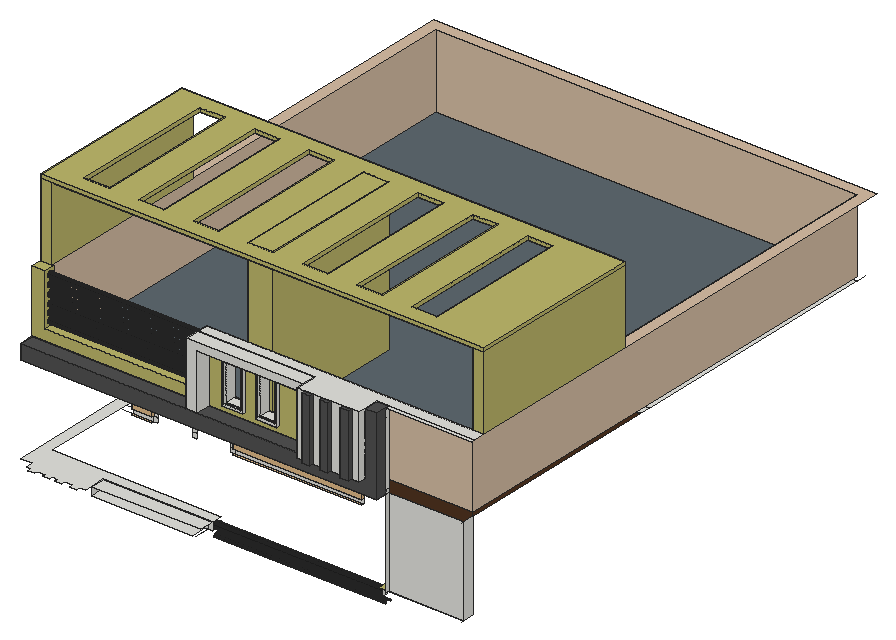
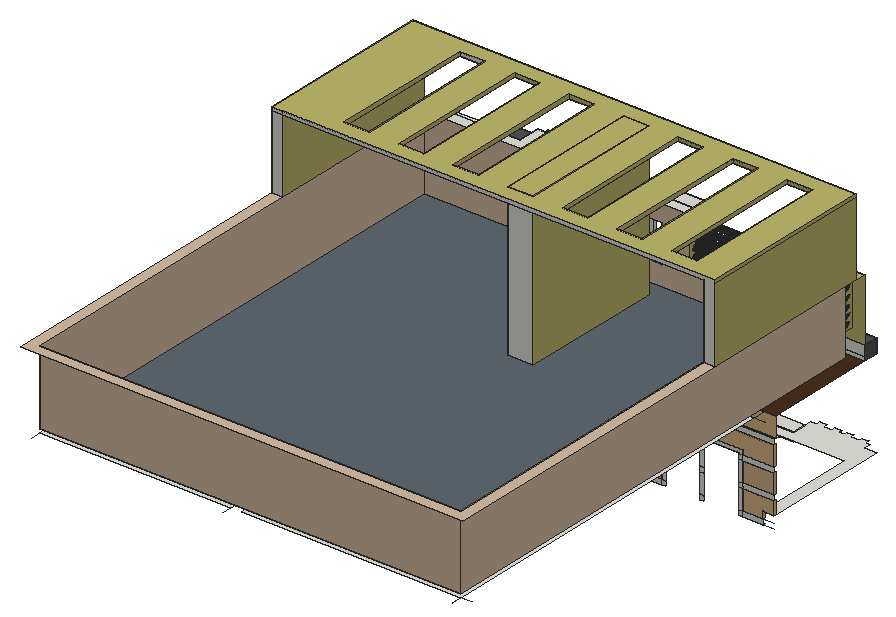
# SketchUp Ruby script. Lengths in inches.
U = 1.inch
M = Sketchup.active_model
def pt(a) = Geom::Point3d.new(a.map { |v| v * U })
def face(e, loops, mat)
  f = e.add_face(loops[0].map { |a| pt(a) })
  loops[1..].each { |l| e.add_face(l.map { |a| pt(a) }).erase! }
  f.material = f.back_material = mat if mat
  f
end
# faces: each face lists its corners as indices into pts; further lists are holes
def faces(e, pts, list, mat = nil) = list.each { |f| face(e, (f[0].is_a?(Array) ? f : [f]).map { |l| l.map { |i| pts[i] } }, mat) }
# xy, xz, yz: faces in a plane at the given z, y or x. An outline is a flat list of corners, or four numbers for a rectangle; further outlines are holes
def ring(l) = l.size == 4 ? [[l[0], l[1]], [l[2], l[1]], [l[2], l[3]], [l[0], l[3]]] : l.each_slice(2).to_a
def flat(e, list, mat, &to3) = list.each { |f| face(e, (f[0].is_a?(Array) ? f : [f]).map { |l| ring(l).map { |u, v| to3.(u, v) } }, mat) }
def xy(e, z, list, mat = nil) = flat(e, list, mat) { |x, y| [x, y, z] }
def xz(e, y, list, mat = nil) = flat(e, list, mat) { |x, z| [x, y, z] }
def yz(e, x, list, mat = nil) = flat(e, list, mat) { |y, z| [x, y, z] }
def lines(e, pts, list) = list.each { |a, b| e.add_line(pt(pts[a]), pt(pts[b])) }
# prism: a flat outline (further loops are holes) pulled along v
def prism(e, loops, v, mat = nil)
  f = face(e, loops, mat); d = Geom::Vector3d.new(v.map { |x| x * U })
  f.pushpull(f.normal.samedirection?(d) ? d.length : -d.length)
end
def box(e, o, s, mat = nil) = prism(e, [[o, [o[0] + s[0], o[1], o[2]], [o[0] + s[0], o[1] + s[1], o[2]], [o[0], o[1] + s[1], o[2]]]], [0, 0, s[2]], mat)
def at(x, y, z, deg = 0) = Geom::Transformation.translation(pt([x, y, z])) * Geom::Transformation.rotation(ORIGIN, Z_AXIS, deg.degrees)
def axes(o, x, y, z) = Geom::Transformation.new([*x, 0, *y, 0, *z, 0, *pt(o).to_a, 1])
def part(name) = M.definitions.add(name)
# library, detail: a bought-in or finely detailed component or shape, given as its bounding box
def library(name, o, s) = part(name).tap { |d| box(d.entities, o, s) }
def detail(e, o, s) = box(e.add_group.entities, o, s)
def put(e, d, t, mat = nil) = e.add_instance(d, t).tap { |i| i.material = mat if mat }
def group(e, t, mat = nil) = e.add_group.tap { |g| g.transformation = t; g.material = mat if mat }.entities
root = M.entities
M.materials.add("[0035_Tan]").color = [210, 180, 140]
M.materials.add("[0036_BurlyWood]").color = [222, 184, 135]
M.materials.add("[0043_SaddleBrown]2").color = [76, 37, 10]
M.materials.add("[0057_DarkKhaki]").color = [189, 183, 107]
M.materials.add("[0135_DarkGray]").color = [81, 81, 81]
M.materials.add("[Beadboard]").color = [71, 46, 29]
M.materials.add("[Blacktop New]").color = [30, 30, 30]
M.materials.add("[Formica Laminate Light]").color = [213, 189, 164]
M.materials.add("[Formica Speckled Grey]").color = [94, 105, 111]
M.materials.add("[Wood Veneer 01]").color = [120, 70, 37]
xy(root,281.25,[[9,110.875,25.44,112.875],[91.44,110.875,195.9375,112.875]],"[0036_BurlyWood]")
xy(root,282.05,[[70.9375,18,88.25,21],[104.5625,18,121.875,21]])
xy(root,284.36,[[57.8125,9,140.4375,21]])
xy(root,285.34,[[9,110.875,25.44,112.875],[91.44,110.875,195.9375,112.875]],"[0036_BurlyWood]")
xy(root,291,[[13.18,0,18.97,0,18.97,3,25.43,3,25.43,0,31.22,0,31.22,3,35.56,3,35.56,0,41.34,0,41.34,3,47.49,3,47.49,0,53.28,0,53.28,3,57.8125,3,57.8125,21,146.625,21,146.625,30,9,30,9,110.875,0,110.875,0,9,9.76,9,9.76,3,13.18,3],[57.8125,9,146.625,21]])
xy(root,291,[[0,110.875,9,112.875]],"[0036_BurlyWood]")
xy(root,291,[[282.375,21,351,30]],"[0057_DarkKhaki]")
xy(root,301.6875,[[0,110.875,9,112.875],[9,110.875,25.44,112.875],[91.44,110.875,195.9375,112.875]],"[0036_BurlyWood]")
xy(root,305.78,[[0,110.875,25.44,112.875]],"[0035_Tan]")
xy(root,305.78,[[91.44,110.875,195.9375,112.875]],"[0036_BurlyWood]")
xy(root,322.125,[[0,110.875,9,112.875],[9,110.875,25.44,112.875]],"[0035_Tan]")
xy(root,322.125,[[91.44,110.875,195.9375,112.875]],"[0036_BurlyWood]")
xy(root,326.22,[[0,110.875,25.44,112.875],[91.44,110.875,195.9375,112.875]],"[0036_BurlyWood]")
xy(root,327,[[28.44,109.875,57.44,112.875],[60.44,109.875,88.44,112.875],[230.67,198,254.61,201],[257.61,198,278.67,201]],"[0043_SaddleBrown]2")
xy(root,330,[[25.44,110.875,91.44,112.875]],"[0036_BurlyWood]")
xy(root,330,[[25.44,109.875,91.44,110.875]],"[0043_SaddleBrown]2")
xy(root,333,[[224.97,200,228.8125,201],[232.16,200,236,201],[239.34,200,243.1875,201],[246.53,200,250.375,201],[253.72,200,257.5625,201],
  [260.91,200,264.75,201],[268.09,200,271.9375,201],[275.28,200,279.125,201],[282.47,200,284.67,201]])
xy(root,333,[[224.67,198,284.67,198,284.67,200,282.47,200,282.47,201,279.125,201,279.125,200,275.28,200,275.28,201,271.9375,201,271.9375,200,268.09,200,268.09,201,264.75,201,264.75,200,260.91,200,260.91,201,257.5625,201,257.5625,200,253.72,200,253.72,201,250.375,201,250.375,200,246.53,200,246.53,201,243.1875,201,243.1875,200,239.34,200,239.34,201,236,201,236,200,232.16,200,232.16,201,228.8125,201,228.8125,200,224.97,200,224.97,201,224.67,201]],"[0043_SaddleBrown]2")
xy(root,342.5625,[[0,110.875,9,112.875],[9,110.875,195.9375,112.875]],"[0036_BurlyWood]")
xy(root,346.66,[[0,110.875,195.9375,112.875]],"[0036_BurlyWood]")
xy(root,363,[[9,121.875,186.9375,420],[196.22,200,200.0625,201],[203.41,200,207.25,201],[210.59,200,214.4375,201],[217.78,200,221.625,201],
  [224.97,200,228.8125,201],[232.16,200,236,201],[239.34,200,243.1875,201],[246.53,200,250.375,201],[253.72,200,257.5625,201],
  [260.91,200,264.75,201],[268.09,200,271.9375,201],[275.28,200,279.125,201],[282.47,200,286.3125,201],[289.66,200,293.5,201],
  [296.84,200,300.6875,201],[304.03,200,307.875,201],[311.22,200,315.0625,201],[318.41,200,322.25,201],[325.59,200,329.4375,201],
  [332.78,200,336.625,201],[339.97,200,343.8125,201],[347.16,200,351,201],[195.9375,201,351,210],[195.9375,210,351,420]])
xy(root,363,[[0,9,290.11,21]],"[0135_DarkGray]")
xy(root,363,[[0,21,0,110.875,195.9375,110.875,195.9375,201,196.22,201,196.22,200,200.0625,200,200.0625,201,203.41,201,203.41,200,207.25,200,207.25,201,210.59,201,210.59,200,214.4375,200,214.4375,201,217.78,201,217.78,200,221.625,200,221.625,201,224.97,201,224.97,200,228.8125,200,228.8125,201,232.16,201,232.16,200,236,200,236,201,239.34,201,239.34,200,243.1875,200,243.1875,201,246.53,201,246.53,200,250.375,200,250.375,201,253.72,201,253.72,200,257.5625,200,257.5625,201,260.91,201,260.91,200,264.75,200,264.75,201,268.09,201,268.09,200,271.9375,200,271.9375,201,275.28,201,275.28,200,279.125,200,279.125,201,282.47,201,282.47,200,286.3125,200,286.3125,201,289.66,201,289.66,200,293.5,200,293.5,201,296.84,201,296.84,200,300.6875,200,300.6875,201,304.03,201,304.03,200,307.875,200,307.875,201,311.22,201,311.22,200,315.0625,200,315.0625,201,318.41,201,318.41,200,322.25,200,322.25,201,325.59,201,325.59,200,329.4375,200,329.4375,201,332.78,201,332.78,200,336.625,200,336.625,201,339.97,201,339.97,200,343.8125,200,343.8125,201,347.16,201,347.16,200,351,200,351,21]],"[Beadboard]")
xy(root,366,[[[9,30,351,420],[157.91,43.02,178.34,160.52]]],"[Formica Speckled Grey]")
xy(root,374.8125,[[229.86,3,280.28,9],[229.86,9,280.28,21]])
xy(root,374.8125,[[235.76,0,242.96,3],[250.32,0,257.52,3],[266.89,0,274.09,3],[0,9,229.86,9,229.86,21,143.76,21,143.76,9.1875,134.73,9.1875,134.73,21,0,21]],"[0135_DarkGray]")
xy(root,379.88,[[155.82,19,173.26,21],[183.51,19,200.94,21]])
xy(root,381.88,[[157.82,19,171.26,21],[185.51,19,198.94,21],[157.82,21,171.26,30],[185.51,21,198.94,30]])
xy(root,384.02,[[10.3125,21,134.73,30]],"[0057_DarkKhaki]")
xy(root,412.81,[[157.82,19,171.26,21],[185.51,19,198.94,21],[157.82,21,171.26,30],[185.51,21,198.94,30]])
xy(root,414.81,[[155.82,19,173.26,21],[183.51,19,200.94,21]])
xy(root,419.8125,[[143.76,9.1875,229.86,21]])
xy(root,426,[[229.86,3,280.28,3,280.28,21,360,21,360,30,134.73,30,134.73,21,229.86,21],[134.73,9.1875,229.86,21],[290.11,18,360,21],[0,30,9,173.11],[351,30,360,173.11]])
xy(root,426,[[0,21,10.3125,30]],"[0057_DarkKhaki]")
xy(root,426,[[235.76,0,242.96,3],[250.32,0,257.52,3],[266.89,0,274.09,3],[280.28,9,290.11,21]],"[0135_DarkGray]")
xy(root,426,[[0,173.11,9,173.11,9,420,351,420,351,173.11,360,173.11,360,429,0,429]],"[Formica Laminate Light]")
xy(root,486,[[351,30,360,173.11]])
xy(root,486,[[[9,30,351,173.11],[113.53,43.02,133.97,160.52],[24.78,43.02,45.22,160.52],[69.16,43.02,89.59,160.52],[202.28,43.02,222.72,160.52],[246.66,43.02,267.09,160.52],[291.03,43.02,311.47,160.52]]],"[0057_DarkKhaki]")
xy(root,489,[[[0,30,360,173.11],[113.53,43.02,133.97,160.52],[24.78,43.02,45.22,160.52],[69.16,43.02,89.59,160.52],[157.91,43.02,178.34,160.52],[202.28,43.02,222.72,160.52],[246.66,43.02,267.09,160.52],[291.03,43.02,311.47,160.52]],[157.91,43.02,178.34,160.52]],"[0057_DarkKhaki]")
xz(root,0,[[235.76,374.8125,242.96,426],[250.32,374.8125,257.52,426],[266.89,374.8125,274.09,426]],"[0135_DarkGray]")
xz(root,3,[[229.86,374.8125,235.76,426],[235.76,374.8125,242.96,426],[242.96,374.8125,250.32,426],[250.32,374.8125,257.52,426],[257.52,374.8125,266.89,426],
  [266.89,374.8125,274.09,426],[274.09,374.8125,280.28,426]])
xz(root,9,[[0,363,290.11,363,290.11,426,280.28,426,280.28,374.8125,0,374.8125]],"[0135_DarkGray]")
xz(root,9.1875,[[134.73,374.8125,143.76,374.8125,143.76,419.8125,229.86,419.8125,229.86,426,134.73,426]])
xz(root,19,[[[155.82,379.88,173.26,414.81],[157.82,381.88,171.26,412.81]],[[183.51,379.88,200.94,414.81],[185.51,381.88,198.94,412.81]]])
xz(root,21,[[57.8125,284.36,142.5625,291],[142.5625,284.36,146.625,291],[290.11,291,351,363],[0,363,290.11,366],[0,366,290.11,366,290.11,426,280.28,426,280.28,374.8125,0,374.8125],
  [134.73,374.8125,143.76,374.8125,143.76,419.8125,229.86,419.8125,229.86,426,134.73,426],[[155.82,379.88,173.26,414.81],[157.82,381.88,171.26,412.81]],[[183.51,379.88,200.94,414.81],[185.51,381.88,198.94,412.81]]])
xz(root,21,[[0,374.8125,134.73,374.8125,134.73,384.02,10.3125,384.02,10.3125,426,0,426],[[143.76,374.8125,229.86,419.8125],[183.51,379.88,200.94,414.81],[155.82,379.88,173.26,414.81]]],"[0057_DarkKhaki]")
xz(root,30,[[0,426,9,486],[351,426,360,486],[0,486,360,489]],"[0057_DarkKhaki]")
xz(root,30,[[[9,366,9,426,10.3125,426,10.3125,384.02,134.73,384.02,134.73,426,351,426,351,366],[185.51,381.88,198.94,412.81],[157.82,381.88,171.26,412.81]]],"[Formica Laminate Light]")
xz(root,43.02,[[291.03,486,311.47,489]])
xz(root,43.02,[[157.91,366,178.34,489],[24.78,486,45.22,489],[69.16,486,89.59,489],[113.53,486,133.97,489],[202.28,486,222.72,489],
  [246.66,486,267.09,489]],"[0057_DarkKhaki]")
xz(root,110.875,[[0,305.78,25.44,322.125]],"[0035_Tan]")
xz(root,110.875,[[9,285.34,25.44,285.34,25.44,301.6875,0,301.6875,0,291,9,291],[91.44,285.34,195.9375,301.6875],[91.44,305.78,195.9375,322.125],[0,326.22,25.44,326.22,25.44,330,91.44,330,91.44,326.22,195.9375,326.22,195.9375,342.5625,0,342.5625],[0,346.66,195.9375,363]],"[0036_BurlyWood]")
xz(root,112.875,[[9,281.25,25.44,285.34],[25.44,281.25,28.44,285.34],[57.44,281.25,60.44,285.34],[88.44,281.25,91.44,285.34],[91.44,281.25,195.9375,285.34],
  [25.44,285.34,28.44,301.6875],[57.44,285.34,60.44,301.6875],[88.44,285.34,91.44,301.6875],[0,301.6875,25.44,305.78],[25.44,301.6875,28.44,305.78],
  [57.44,301.6875,60.44,305.78],[88.44,301.6875,91.44,305.78],[91.44,301.6875,195.9375,305.78],[25.44,305.78,28.44,322.125],[57.44,305.78,60.44,322.125],
  [88.44,305.78,91.44,322.125],[0,322.125,25.44,326.22],[25.44,322.125,28.44,326.22],[57.44,322.125,60.44,326.22],[88.44,322.125,91.44,326.22],
  [91.44,322.125,195.9375,326.22],[25.44,326.22,28.44,326.22,28.44,327,57.44,327,57.44,326.22,60.44,326.22,60.44,327,88.44,327,88.44,326.22,91.44,326.22,91.44,330,25.44,330],[0,342.5625,195.9375,346.66]])
xz(root,112.875,[[0,305.78,25.44,322.125]],"[0035_Tan]")
xz(root,112.875,[[9,285.34,9,291,0,291,0,301.6875,25.44,301.6875,25.44,285.34],[91.44,285.34,195.9375,301.6875],[91.44,305.78,195.9375,322.125],[0,326.22,0,342.5625,195.9375,342.5625,195.9375,326.22,91.44,326.22,91.44,330,25.44,330,25.44,326.22]],"[0036_BurlyWood]")
xz(root,160.52,[[157.91,366,178.34,489]])
xz(root,160.52,[[24.78,486,45.22,489],[69.16,486,89.59,489],[113.53,486,133.97,489],[202.28,486,222.72,489],[246.66,486,267.09,489],
  [291.03,486,311.47,489]],"[0057_DarkKhaki]")
xz(root,173.11,[[0,426,0,489,351,489,351,486,9,486,9,426],[351,426,360,486],[351,486,360,489]])
xz(root,200,[[224.97,333,228.8125,363],[232.16,333,236,363],[239.34,333,243.1875,363],[246.53,333,250.375,363],[253.72,333,257.5625,363],
  [260.91,333,264.75,363],[268.09,333,271.9375,363],[275.28,333,279.125,363]],"[Wood Veneer 01]")
xz(root,201,[[232.16,327,236,333],[236,327,239.34,333],[239.34,327,243.1875,333],[243.1875,327,246.53,333],[246.53,327,250.375,333],
  [250.375,327,253.72,333],[260.91,327,264.75,333],[264.75,327,268.09,333],[268.09,327,271.9375,333],[271.9375,327,275.28,333],
  [224.97,333,228.8125,363],[232.16,333,236,363],[239.34,333,243.1875,363],[246.53,333,250.375,363],[253.72,333,257.5625,363],
  [260.91,333,264.75,363],[268.09,333,271.9375,363],[275.28,333,279.125,363]])
xz(root,201,[[228.8125,333,232.16,363],[236,333,239.34,363],[243.1875,333,246.53,363],[250.375,333,253.72,363],[257.5625,333,260.91,363],
  [264.75,333,268.09,363],[271.9375,333,275.28,363],[279.125,333,282.47,363]],"[Wood Veneer 01]")
xz(root,420,[[9,366,351,426]],"[Formica Laminate Light]")
yz(root,0,[[110.875,305.78,112.875,322.125]],"[0035_Tan]")
yz(root,0,[[110.875,291,112.875,301.6875],[110.875,326.22,112.875,342.5625]],"[0036_BurlyWood]")
yz(root,0,[[30,426,173.11,486],[30,486,173.11,489]],"[0057_DarkKhaki]")
yz(root,0,[[9,363,21,374.8125]],"[0135_DarkGray]")
yz(root,9,[[110.875,285.34,112.875,291]],"[0036_BurlyWood]")
yz(root,9,[[30,426,173.11,486]],"[0057_DarkKhaki]")
yz(root,9,[[30,366,420,426]],"[Formica Laminate Light]")
yz(root,10.3125,[[[21,384.02,30,426],[25.41,412.65,24.83,412.73,24.29,412.95,23.82,413.3125,23.46,413.78,23.24,414.32,23.16,414.9,23.24,415.48,23.46,416.03,23.82,416.49,24.29,416.85,24.83,417.08,25.41,417.15,25.99,417.08,26.54,416.85,27,416.49,27.36,416.03,27.59,415.48,27.66,414.9,27.59,414.32,27.36,413.78,27,413.3125,26.54,412.95,25.99,412.73],[25.41,405.59,24.83,405.67,24.29,405.89,23.82,406.25,23.46,406.71,23.24,407.26,23.16,407.84,23.24,408.42,23.46,408.96,23.82,409.43,24.29,409.79,24.83,410.01,25.41,410.09,25.99,410.01,26.54,409.79,27,409.43,27.36,408.96,27.59,408.42,27.66,407.84,27.59,407.26,27.36,406.71,27,406.25,26.54,405.89,25.99,405.67],[25.41,398.53,24.83,398.6,24.29,398.83,23.82,399.1875,23.46,399.65,23.24,400.19,23.16,400.78,23.24,401.36,23.46,401.9,23.82,402.37,24.29,402.73,24.83,402.95,25.41,403.03,25.99,402.95,26.54,402.73,27,402.37,27.36,401.9,27.59,401.36,27.66,400.78,27.59,400.19,27.36,399.65,27,399.1875,26.54,398.83,25.99,398.6],[25.41,392.4,24.83,392.48,24.29,392.7,23.82,393.0625,23.46,393.53,23.24,394.07,23.16,394.65,23.24,395.23,23.46,395.78,23.82,396.24,24.29,396.6,24.83,396.83,25.41,396.9,25.99,396.83,26.54,396.6,27,396.24,27.36,395.78,27.59,395.23,27.66,394.65,27.59,394.07,27.36,393.53,27,393.0625,26.54,392.7,25.99,392.48],[25.41,386.21,24.83,386.29,24.29,386.52,23.82,386.875,23.46,387.34,23.24,387.88,23.16,388.46,23.24,389.05,23.46,389.59,23.82,390.06,24.29,390.41,24.83,390.64,25.41,390.71,25.99,390.64,26.54,390.41,27,390.06,27.36,389.59,27.59,389.05,27.66,388.46,27.59,387.88,27.36,387.34,27,386.875,26.54,386.52,25.99,386.29],[25.41,419.71,24.83,419.79,24.29,420.02,23.82,420.375,23.46,420.84,23.24,421.38,23.16,421.96,23.24,422.55,23.46,423.09,23.82,423.56,24.29,423.91,24.83,424.14,25.41,424.21,25.99,424.14,26.54,423.91,27,423.56,27.36,423.09,27.59,422.55,27.66,421.96,27.59,421.38,27.36,420.84,27,420.375,26.54,420.02,25.99,419.79]]],"[0057_DarkKhaki]")
yz(root,24.78,[[43.02,486,160.52,489]],"[0057_DarkKhaki]")
yz(root,25.44,[[110.875,305.78,112.875,322.125]],"[0035_Tan]")
yz(root,25.44,[[110.875,285.34,112.875,301.6875],[110.875,326.22,112.875,330]],"[0036_BurlyWood]")
yz(root,45.22,[[43.02,486,160.52,489]],"[0057_DarkKhaki]")
yz(root,57.8125,[[9,284.36,21,291]])
yz(root,69.16,[[43.02,486,160.52,489]],"[0057_DarkKhaki]")
yz(root,89.59,[[43.02,486,160.52,489]],"[0057_DarkKhaki]")
yz(root,91.44,[[110.875,285.34,112.875,301.6875],[110.875,305.78,112.875,322.125],[110.875,326.22,112.875,330]],"[0036_BurlyWood]")
yz(root,113.53,[[43.02,486,160.52,489]],"[0057_DarkKhaki]")
yz(root,133.97,[[43.02,486,160.52,489]],"[0057_DarkKhaki]")
yz(root,134.73,[[9.1875,374.8125,21,426]])
yz(root,134.73,[[[21,384.02,30,426],[25.41,386.21,25.99,386.29,26.54,386.52,27,386.875,27.36,387.34,27.59,387.88,27.66,388.46,27.59,389.05,27.36,389.59,27,390.06,26.54,390.41,25.99,390.64,25.41,390.71,24.83,390.64,24.29,390.41,23.82,390.06,23.46,389.59,23.24,389.05,23.16,388.46,23.24,387.88,23.46,387.34,23.82,386.875,24.29,386.52,24.83,386.29],[25.41,392.4,25.99,392.48,26.54,392.7,27,393.0625,27.36,393.53,27.59,394.07,27.66,394.65,27.59,395.23,27.36,395.78,27,396.24,26.54,396.6,25.99,396.83,25.41,396.9,24.83,396.83,24.29,396.6,23.82,396.24,23.46,395.78,23.24,395.23,23.16,394.65,23.24,394.07,23.46,393.53,23.82,393.0625,24.29,392.7,24.83,392.48],[25.41,398.53,25.99,398.6,26.54,398.83,27,399.1875,27.36,399.65,27.59,400.19,27.66,400.78,27.59,401.36,27.36,401.9,27,402.37,26.54,402.73,25.99,402.95,25.41,403.03,24.83,402.95,24.29,402.73,23.82,402.37,23.46,401.9,23.24,401.36,23.16,400.78,23.24,400.19,23.46,399.65,23.82,399.1875,24.29,398.83,24.83,398.6],[25.41,412.65,25.99,412.73,26.54,412.95,27,413.3125,27.36,413.78,27.59,414.32,27.66,414.9,27.59,415.48,27.36,416.03,27,416.49,26.54,416.85,25.99,417.08,25.41,417.15,24.83,417.08,24.29,416.85,23.82,416.49,23.46,416.03,23.24,415.48,23.16,414.9,23.24,414.32,23.46,413.78,23.82,413.3125,24.29,412.95,24.83,412.73],[25.41,419.71,25.99,419.79,26.54,420.02,27,420.375,27.36,420.84,27.59,421.38,27.66,421.96,27.59,422.55,27.36,423.09,27,423.56,26.54,423.91,25.99,424.14,25.41,424.21,24.83,424.14,24.29,423.91,23.82,423.56,23.46,423.09,23.24,422.55,23.16,421.96,23.24,421.38,23.46,420.84,23.82,420.375,24.29,420.02,24.83,419.79]]],"[0057_DarkKhaki]")
yz(root,138.5625,[[25.41,405.59,25.99,405.67,26.54,405.89,27,406.25,27.36,406.71,27.59,407.26,27.66,407.84,27.59,408.42,27.36,408.96,27,409.43,26.54,409.79,25.99,410.01,25.41,410.09,24.83,410.01,24.29,409.79,23.82,409.43,23.46,408.96,23.24,408.42,23.16,407.84,23.24,407.26,23.46,406.71,23.82,406.25,24.29,405.89,24.83,405.67]])
yz(root,143.76,[[9.1875,374.8125,21,419.8125]])
yz(root,155.82,[[19,379.88,21,414.81]])
yz(root,157.82,[[19,381.88,21,412.81],[21,381.88,30,412.81]])
yz(root,157.91,[[43.02,366,160.52,489]],"[0057_DarkKhaki]")
yz(root,171.26,[[19,381.88,21,412.81],[21,381.88,30,412.81]])
yz(root,173.26,[[19,379.88,21,414.81]])
yz(root,178.34,[[43.02,366,160.52,489]],"[0057_DarkKhaki]")
yz(root,183.51,[[19,379.88,21,414.81]])
yz(root,185.51,[[19,381.88,21,412.81],[21,381.88,30,412.81]])
yz(root,195.9375,[[110.875,285.34,112.875,301.6875],[110.875,305.78,112.875,322.125],[110.875,326.22,112.875,342.5625]],"[0036_BurlyWood]")
yz(root,198.94,[[19,381.88,21,412.81],[21,381.88,30,412.81]])
yz(root,200.94,[[19,379.88,21,414.81]])
yz(root,202.28,[[43.02,486,160.52,489]],"[0057_DarkKhaki]")
yz(root,222.72,[[43.02,486,160.52,489]],"[0057_DarkKhaki]")
yz(root,224.97,[[200,333,201,363]])
yz(root,228.8125,[[200,333,201,363]],"[Wood Veneer 01]")
yz(root,229.86,[[3,374.8125,3,426,9.1875,426,9.1875,419.8125,21,419.8125,21,374.8125],[9.1875,419.8125,21,426]])
yz(root,232.16,[[200,333,201,363]])
yz(root,235.76,[[0,374.8125,3,426]],"[0135_DarkGray]")
yz(root,236,[[200,333,201,363]],"[Wood Veneer 01]")
yz(root,239.34,[[200,333,201,363]])
yz(root,242.96,[[0,374.8125,3,426]],"[0135_DarkGray]")
yz(root,243.1875,[[200,333,201,363]],"[Wood Veneer 01]")
yz(root,246.53,[[200,333,201,363]])
yz(root,246.66,[[43.02,486,160.52,489]],"[0057_DarkKhaki]")
yz(root,250.32,[[0,374.8125,3,426]],"[0135_DarkGray]")
yz(root,250.375,[[200,333,201,363]])
yz(root,253.72,[[200,333,201,363]])
yz(root,257.52,[[0,374.8125,3,426]],"[0135_DarkGray]")
yz(root,257.5625,[[200,333,201,363]])
yz(root,260.91,[[200,333,201,363]])
yz(root,264.75,[[200,333,201,363]])
yz(root,266.89,[[0,374.8125,3,426]],"[0135_DarkGray]")
yz(root,267.09,[[43.02,486,160.52,489]],"[0057_DarkKhaki]")
yz(root,268.09,[[200,333,201,363]])
yz(root,271.9375,[[200,333,201,363]])
yz(root,274.09,[[0,374.8125,3,426]],"[0135_DarkGray]")
yz(root,275.28,[[200,333,201,363]])
yz(root,279.125,[[200,333,201,363]])
yz(root,280.28,[[3,374.8125,9,426],[9,374.8125,21,426]])
yz(root,282.47,[[200,333,201,363]])
yz(root,283.6875,[[25.25,284.3125,25.99,284.41,26.68,284.7,27.28,285.15,27.74,285.75,28.02,286.44,28.12,287.1875,28.02,287.93,27.74,288.625,27.28,289.22,26.68,289.68,25.99,289.96,25.25,290.0625,24.5,289.96,23.81,289.68,23.21,289.22,22.76,288.625,22.47,287.93,22.37,287.1875,22.47,286.44,22.76,285.75,23.21,285.15,23.81,284.7,24.5,284.41]])
yz(root,290.11,[[18,291,21,363],[18,363,21,366],[18,366,21,426]])
yz(root,290.11,[[9,363,18,426]],"[0135_DarkGray]")
yz(root,291.03,[[43.02,486,160.52,489]],"[0057_DarkKhaki]")
yz(root,311.47,[[43.02,486,160.52,489]],"[0057_DarkKhaki]")
yz(root,351,[[21,291,30,363]])
yz(root,351,[[30,426,173.11,486]],"[0057_DarkKhaki]")
yz(root,351,[[30,366,420,426]],"[Formica Laminate Light]")
yz(root,360,[[30,426,173.11,486],[30,486,173.11,489]],"[0057_DarkKhaki]")
p = [[146.625,22.76,280.3125],[146.625,22.47,279.62],[286.1875,22.47,279.62],[286.1875,22.76,280.3125],[146.625,28.02,279.62],[146.625,27.74,280.3125],
  [286.1875,27.74,280.3125],[286.1875,28.02,279.62],[146.625,23.21,280.91],[286.1875,23.21,280.91],[146.625,27.28,280.91],[286.1875,27.28,280.91],
  [146.625,23.81,281.37],[286.1875,23.81,281.37],[146.625,26.68,281.37],[286.1875,26.68,281.37],[146.625,24.5,281.65],[286.1875,24.5,281.65],
  [146.625,25.99,281.65],[286.1875,25.99,281.65],[146.625,25.25,281.75],[286.1875,25.25,281.75],[146.625,24.5,284.41],[146.625,25.25,284.3125],
  [283.6875,25.25,284.3125],[283.6875,24.5,284.41],[146.625,25.99,284.41],[283.6875,25.99,284.41],[146.625,23.81,284.7],[283.6875,23.81,284.7],
  [146.625,26.68,284.7],[283.6875,26.68,284.7],[146.625,23.21,285.15],[283.6875,23.21,285.15],[146.625,27.28,285.15],[283.6875,27.28,285.15],
  [146.625,22.76,285.75],[283.6875,22.76,285.75],[146.625,27.74,285.75],[283.6875,27.74,285.75],[146.625,22.47,286.44],[283.6875,22.47,286.44],
  [146.625,28.02,286.44],[283.6875,28.02,286.44],[146.625,22.37,287.1875],[283.6875,22.37,287.1875],[146.625,28.12,287.1875],[283.6875,28.12,287.1875],
  [146.625,22.47,287.93],[283.6875,22.47,287.93],[146.625,28.02,287.93],[283.6875,28.02,287.93],[146.625,22.76,288.625],[283.6875,22.76,288.625],
  [146.625,27.74,288.625],[283.6875,27.74,288.625],[146.625,23.21,289.22],[283.6875,23.21,289.22],[146.625,27.28,289.22],[283.6875,27.28,289.22],
  [146.625,23.81,289.68],[283.6875,23.81,289.68],[146.625,26.68,289.68],[283.6875,26.68,289.68],[146.625,24.5,289.96],[283.6875,24.5,289.96],
  [146.625,25.99,289.96],[283.6875,25.99,289.96],[146.625,25.25,290.0625],[283.6875,25.25,290.0625],[10.3125,24.83,386.29],[10.3125,25.41,386.21],
  [134.73,25.41,386.21],[134.73,24.83,386.29],[10.3125,25.99,386.29],[134.73,25.99,386.29],[10.3125,24.29,386.52],[134.73,24.29,386.52],
  [10.3125,26.54,386.52],[134.73,26.54,386.52],[10.3125,23.82,386.875],[134.73,23.82,386.875],[10.3125,27,386.875],[134.73,27,386.875],
  [10.3125,23.46,387.34],[134.73,23.46,387.34],[10.3125,27.36,387.34],[134.73,27.36,387.34],[10.3125,23.24,387.88],[134.73,23.24,387.88],
  [10.3125,27.59,387.88],[134.73,27.59,387.88],[10.3125,23.16,388.46],[134.73,23.16,388.46],[10.3125,27.66,388.46],[134.73,27.66,388.46],
  [10.3125,23.24,389.05],[134.73,23.24,389.05],[10.3125,27.59,389.05],[134.73,27.59,389.05],[10.3125,23.46,389.59],[134.73,23.46,389.59],
  [10.3125,27.36,389.59],[134.73,27.36,389.59],[10.3125,23.82,390.06],[134.73,23.82,390.06],[10.3125,27,390.06],[134.73,27,390.06],
  [10.3125,24.29,390.41],[134.73,24.29,390.41],[10.3125,26.54,390.41],[134.73,26.54,390.41],[10.3125,24.83,390.64],[134.73,24.83,390.64],
  [10.3125,25.99,390.64],[134.73,25.99,390.64],[10.3125,25.41,390.71],[134.73,25.41,390.71],[10.3125,24.83,392.48],[10.3125,25.41,392.4],
  [134.73,25.41,392.4],[134.73,24.83,392.48],[10.3125,25.99,392.48],[134.73,25.99,392.48],[10.3125,24.29,392.7],[134.73,24.29,392.7],
  [10.3125,26.54,392.7],[134.73,26.54,392.7],[10.3125,23.82,393.0625],[134.73,23.82,393.0625],[10.3125,27,393.0625],[134.73,27,393.0625],
  [10.3125,23.46,393.53],[134.73,23.46,393.53],[10.3125,27.36,393.53],[134.73,27.36,393.53],[10.3125,23.24,394.07],[134.73,23.24,394.07],
  [10.3125,27.59,394.07],[134.73,27.59,394.07],[10.3125,23.16,394.65],[134.73,23.16,394.65],[10.3125,27.66,394.65],[134.73,27.66,394.65],
  [10.3125,23.24,395.23],[134.73,23.24,395.23],[10.3125,27.59,395.23],[134.73,27.59,395.23],[10.3125,23.46,395.78],[134.73,23.46,395.78],
  [10.3125,27.36,395.78],[134.73,27.36,395.78],[10.3125,23.82,396.24],[134.73,23.82,396.24],[10.3125,27,396.24],[134.73,27,396.24],
  [10.3125,24.29,396.6],[134.73,24.29,396.6],[10.3125,26.54,396.6],[134.73,26.54,396.6],[10.3125,24.83,396.83],[134.73,24.83,396.83],
  [10.3125,25.99,396.83],[134.73,25.99,396.83],[10.3125,25.41,396.9],[134.73,25.41,396.9],[10.3125,24.83,398.6],[10.3125,25.41,398.53],
  [134.73,25.41,398.53],[134.73,24.83,398.6],[10.3125,25.99,398.6],[134.73,25.99,398.6],[10.3125,24.29,398.83],[134.73,24.29,398.83],
  [10.3125,26.54,398.83],[134.73,26.54,398.83],[10.3125,23.82,399.1875],[134.73,23.82,399.1875],[10.3125,27,399.1875],[134.73,27,399.1875],
  [10.3125,23.46,399.65],[134.73,23.46,399.65],[10.3125,27.36,399.65],[134.73,27.36,399.65],[10.3125,23.24,400.19],[134.73,23.24,400.19],
  [10.3125,27.59,400.19],[134.73,27.59,400.19],[10.3125,23.16,400.78],[134.73,23.16,400.78],[10.3125,27.66,400.78],[134.73,27.66,400.78],
  [10.3125,23.24,401.36],[134.73,23.24,401.36],[10.3125,27.59,401.36],[134.73,27.59,401.36],[10.3125,23.46,401.9],[134.73,23.46,401.9],
  [10.3125,27.36,401.9],[134.73,27.36,401.9],[10.3125,23.82,402.37],[134.73,23.82,402.37],[10.3125,27,402.37],[134.73,27,402.37],
  [10.3125,24.29,402.73],[134.73,24.29,402.73],[10.3125,26.54,402.73],[134.73,26.54,402.73],[10.3125,24.83,402.95],[134.73,24.83,402.95],
  [10.3125,25.99,402.95],[134.73,25.99,402.95],[10.3125,25.41,403.03],[134.73,25.41,403.03],[10.3125,24.83,405.67],[10.3125,25.41,405.59],
  [138.5625,25.41,405.59],[138.5625,24.83,405.67],[10.3125,25.99,405.67],[138.5625,25.99,405.67],[10.3125,24.29,405.89],[138.5625,24.29,405.89],
  [10.3125,26.54,405.89],[138.5625,26.54,405.89],[10.3125,23.82,406.25],[138.5625,23.82,406.25],[10.3125,27,406.25],[138.5625,27,406.25],
  [10.3125,23.46,406.71],[138.5625,23.46,406.71],[10.3125,27.36,406.71],[138.5625,27.36,406.71],[10.3125,23.24,407.26],[138.5625,23.24,407.26],
  [10.3125,27.59,407.26],[138.5625,27.59,407.26],[10.3125,23.16,407.84],[138.5625,23.16,407.84],[10.3125,27.66,407.84],[138.5625,27.66,407.84],
  [10.3125,23.24,408.42],[138.5625,23.24,408.42],[10.3125,27.59,408.42],[138.5625,27.59,408.42],[10.3125,23.46,408.96],[138.5625,23.46,408.96],
  [10.3125,27.36,408.96],[138.5625,27.36,408.96],[10.3125,23.82,409.43],[138.5625,23.82,409.43],[10.3125,27,409.43],[138.5625,27,409.43],
  [10.3125,24.29,409.79],[138.5625,24.29,409.79],[10.3125,26.54,409.79],[138.5625,26.54,409.79],[10.3125,24.83,410.01],[138.5625,24.83,410.01],
  [10.3125,25.99,410.01],[138.5625,25.99,410.01],[10.3125,25.41,410.09],[138.5625,25.41,410.09],[10.3125,24.29,412.95],[10.3125,24.83,412.73],
  [134.73,24.83,412.73],[134.73,24.29,412.95],[10.3125,25.41,412.65],[134.73,25.41,412.65],[10.3125,25.99,412.73],[134.73,25.99,412.73],
  [10.3125,26.54,412.95],[134.73,26.54,412.95],[10.3125,23.82,413.3125],[134.73,23.82,413.3125],[10.3125,27,413.3125],[134.73,27,413.3125],
  [10.3125,23.46,413.78],[134.73,23.46,413.78],[10.3125,27.36,413.78],[134.73,27.36,413.78],[10.3125,23.24,414.32],[134.73,23.24,414.32],
  [10.3125,27.59,414.32],[134.73,27.59,414.32],[10.3125,23.16,414.9],[134.73,23.16,414.9],[10.3125,27.66,414.9],[134.73,27.66,414.9],
  [10.3125,23.24,415.48],[134.73,23.24,415.48],[10.3125,27.59,415.48],[134.73,27.59,415.48],[10.3125,23.46,416.03],[134.73,23.46,416.03],
  [10.3125,27.36,416.03],[134.73,27.36,416.03],[10.3125,23.82,416.49],[134.73,23.82,416.49],[10.3125,27,416.49],[134.73,27,416.49],
  [10.3125,24.29,416.85],[134.73,24.29,416.85],[10.3125,26.54,416.85],[134.73,26.54,416.85],[10.3125,24.83,417.08],[134.73,24.83,417.08],
  [10.3125,25.99,417.08],[134.73,25.99,417.08],[10.3125,25.41,417.15],[134.73,25.41,417.15],[10.3125,24.83,419.79],[10.3125,25.41,419.71],
  [134.73,25.41,419.71],[134.73,24.83,419.79],[10.3125,25.99,419.79],[134.73,25.99,419.79],[10.3125,24.29,420.02],[134.73,24.29,420.02],
  [10.3125,26.54,420.02],[134.73,26.54,420.02],[10.3125,23.82,420.375],[134.73,23.82,420.375],[10.3125,27,420.375],[134.73,27,420.375],
  [10.3125,23.46,420.84],[134.73,23.46,420.84],[10.3125,27.36,420.84],[134.73,27.36,420.84],[10.3125,23.24,421.38],[134.73,23.24,421.38],
  [10.3125,27.59,421.38],[134.73,27.59,421.38],[10.3125,23.16,421.96],[134.73,23.16,421.96],[10.3125,27.66,421.96],[134.73,27.66,421.96],
  [10.3125,23.24,422.55],[134.73,23.24,422.55],[10.3125,27.59,422.55],[134.73,27.59,422.55],[10.3125,23.46,423.09],[134.73,23.46,423.09],
  [10.3125,27.36,423.09],[134.73,27.36,423.09],[10.3125,23.82,423.56],[134.73,23.82,423.56],[10.3125,27,423.56],[134.73,27,423.56],
  [10.3125,24.29,423.91],[134.73,24.29,423.91],[10.3125,26.54,423.91],[134.73,26.54,423.91],[10.3125,24.83,424.14],[134.73,24.83,424.14],
  [10.3125,25.99,424.14],[134.73,25.99,424.14],[10.3125,25.41,424.21],[134.73,25.41,424.21],[351,420,363],[351,429,363],
  [351,30,363],[351,30,366],[9,112.875,363],[9,112.875,366],[9,121.875,363],[9,420,363],
  [9,429,363],[195.9375,420,363],[195.9375,429,363],[0,420,363],[0,121.875,363],[142.5625,21,284.36],
  [142.5625,9,284.36],[9,112.875,285.34],[0,112.875,285.34],[0,112.875,281.25],[9,112.875,281.25],[351,21,291],
  [351,18,291],[351,21,363],[351,18,363],[195.9375,112.875,363],[195.9375,112.875,366]]
faces(root,p,[[0,1,2,3],[4,5,6,7],[8,0,3,9],[5,10,11,6],[12,8,9,13],[10,14,15,11],[16,12,13,17],[14,18,19,15],
  [20,16,17,21],[18,20,21,19],[22,23,24,25],[23,26,27,24],[28,22,25,29],[26,30,31,27],[32,28,29,33],[30,34,35,31],
  [36,32,33,37],[34,38,39,35],[40,36,37,41],[38,42,43,39],[44,40,41,45],[42,46,47,43],[48,44,45,49],[46,50,51,47],
  [52,48,49,53],[50,54,55,51],[56,52,53,57],[54,58,59,55],[60,56,57,61],[58,62,63,59],[64,60,61,65],[62,66,67,63],
  [68,64,65,69],[66,68,69,67],[70,71,72,73],[71,74,75,72],[76,70,73,77],[74,78,79,75],[80,76,77,81],[78,82,83,79],
  [84,80,81,85],[82,86,87,83],[88,84,85,89],[86,90,91,87],[92,88,89,93],[90,94,95,91],[96,92,93,97],[94,98,99,95],
  [100,96,97,101],[98,102,103,99],[104,100,101,105],[102,106,107,103],[108,104,105,109],[106,110,111,107],[112,108,109,113],[110,114,115,111],
  [116,112,113,117],[114,116,117,115],[118,119,120,121],[119,122,123,120],[124,118,121,125],[122,126,127,123],[128,124,125,129],[126,130,131,127],
  [132,128,129,133],[130,134,135,131],[136,132,133,137],[134,138,139,135],[140,136,137,141],[138,142,143,139],[144,140,141,145],[142,146,147,143],
  [148,144,145,149],[146,150,151,147],[152,148,149,153],[150,154,155,151],[156,152,153,157],[154,158,159,155],[160,156,157,161],[158,162,163,159],
  [164,160,161,165],[162,164,165,163],[166,167,168,169],[167,170,171,168],[172,166,169,173],[170,174,175,171],[176,172,173,177],[174,178,179,175],
  [180,176,177,181],[178,182,183,179],[184,180,181,185],[182,186,187,183],[188,184,185,189],[186,190,191,187],[192,188,189,193],[190,194,195,191],
  [196,192,193,197],[194,198,199,195],[200,196,197,201],[198,202,203,199],[204,200,201,205],[202,206,207,203],[208,204,205,209],[206,210,211,207],
  [212,208,209,213],[210,212,213,211],[214,215,216,217],[215,218,219,216],[220,214,217,221],[218,222,223,219],[224,220,221,225],[222,226,227,223],
  [228,224,225,229],[226,230,231,227],[232,228,229,233],[230,234,235,231],[236,232,233,237],[234,238,239,235],[240,236,237,241],[238,242,243,239],
  [244,240,241,245],[242,246,247,243],[248,244,245,249],[246,250,251,247],[252,248,249,253],[250,254,255,251],[256,252,253,257],[254,258,259,255],
  [260,256,257,261],[258,260,261,259],[262,263,264,265],[263,266,267,264],[266,268,269,267],[268,270,271,269],[272,262,265,273],[270,274,275,271],
  [276,272,273,277],[274,278,279,275],[280,276,277,281],[278,282,283,279],[284,280,281,285],[282,286,287,283],[288,284,285,289],[286,290,291,287],
  [292,288,289,293],[290,294,295,291],[296,292,293,297],[294,298,299,295],[300,296,297,301],[298,302,303,299],[304,300,301,305],[302,306,307,303],
  [308,304,305,309],[306,308,309,307],[310,311,312,313],[311,314,315,312],[316,310,313,317],[314,318,319,315],[320,316,317,321],[318,322,323,319],
  [324,320,321,325],[322,326,327,323],[328,324,325,329],[326,330,331,327],[332,328,329,333],[330,334,335,331],[336,332,333,337],[334,338,339,335],
  [340,336,337,341],[338,342,343,339],[344,340,341,345],[342,346,347,343],[348,344,345,349],[346,350,351,347],[352,348,349,353],[350,354,355,351],
  [356,352,353,357],[354,356,357,355]],"[Blacktop New]")
lines(root,p,[[358,359],[360,361],[362,363],[362,364],[365,366],[367,368],[365,369],[364,370],[371,372],[373,374],[375,376],[377,378],
  [379,380],[381,382]])
